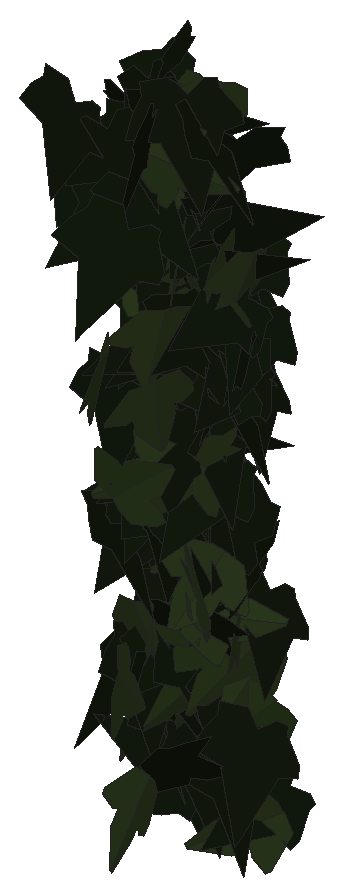
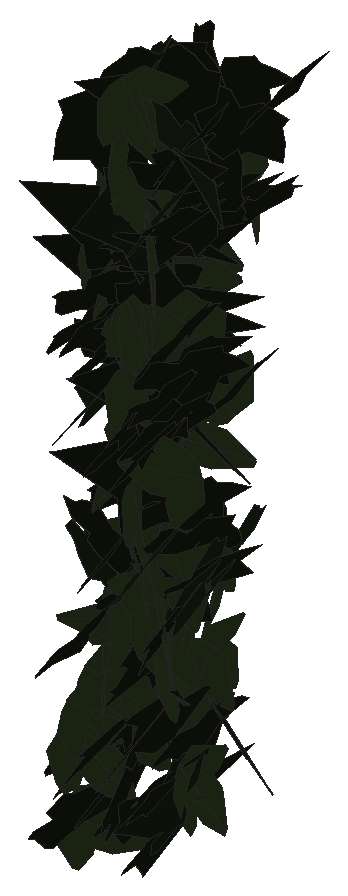
# SketchUp Ruby script. Lengths in inches.
U = 1.inch
M = Sketchup.active_model
def pt(a) = Geom::Point3d.new(a.map { |v| v * U })
def face(e, loops, mat)
  f = e.add_face(loops[0].map { |a| pt(a) })
  loops[1..].each { |l| e.add_face(l.map { |a| pt(a) }).erase! }
  f.material = f.back_material = mat if mat
  f
end
# faces: each face lists its corners as indices into pts; further lists are holes
def faces(e, pts, list, mat = nil) = list.each { |f| face(e, (f[0].is_a?(Array) ? f : [f]).map { |l| l.map { |i| pts[i] } }, mat) }
# xy, xz, yz: faces in a plane at the given z, y or x. An outline is a flat list of corners, or four numbers for a rectangle; further outlines are holes
def ring(l) = l.size == 4 ? [[l[0], l[1]], [l[2], l[1]], [l[2], l[3]], [l[0], l[3]]] : l.each_slice(2).to_a
def flat(e, list, mat, &to3) = list.each { |f| face(e, (f[0].is_a?(Array) ? f : [f]).map { |l| ring(l).map { |u, v| to3.(u, v) } }, mat) }
def xy(e, z, list, mat = nil) = flat(e, list, mat) { |x, y| [x, y, z] }
def xz(e, y, list, mat = nil) = flat(e, list, mat) { |x, z| [x, y, z] }
def yz(e, x, list, mat = nil) = flat(e, list, mat) { |y, z| [x, y, z] }
def lines(e, pts, list) = list.each { |a, b| e.add_line(pt(pts[a]), pt(pts[b])) }
# prism: a flat outline (further loops are holes) pulled along v
def prism(e, loops, v, mat = nil)
  f = face(e, loops, mat); d = Geom::Vector3d.new(v.map { |x| x * U })
  f.pushpull(f.normal.samedirection?(d) ? d.length : -d.length)
end
def box(e, o, s, mat = nil) = prism(e, [[o, [o[0] + s[0], o[1], o[2]], [o[0] + s[0], o[1] + s[1], o[2]], [o[0], o[1] + s[1], o[2]]]], [0, 0, s[2]], mat)
def at(x, y, z, deg = 0) = Geom::Transformation.translation(pt([x, y, z])) * Geom::Transformation.rotation(ORIGIN, Z_AXIS, deg.degrees)
def axes(o, x, y, z) = Geom::Transformation.new([*x, 0, *y, 0, *z, 0, *pt(o).to_a, 1])
def part(name) = M.definitions.add(name)
# library, detail: a bought-in or finely detailed component or shape, given as its bounding box
def library(name, o, s) = part(name).tap { |d| box(d.entities, o, s) }
def detail(e, o, s) = box(e.add_group.entities, o, s)
def put(e, d, t, mat = nil) = e.add_instance(d, t).tap { |i| i.material = mat if mat }
def group(e, t, mat = nil) = e.add_group.tap { |g| g.transformation = t; g.material = mat if mat }.entities
root = M.entities
M.materials.add("efeu1").color = [18, 25, 13]
M.materials.add("efeu2").color = [43, 57, 29]
c1 = part("ivyleaf_9")
p = [[1.54,2.16,1.25],[1.36,2.04,1.19],[-0.21,0.99,0.68],[-0.71,1.11,0.82],[-0.85,0.86,0.67],[-0.8,0.17,0.21],
  [-0.9,-0.01,0.1],[-0.67,-0.16,-0.02],[-0.08,-0.08,-0.05],[-0.03,-0.6,-0.4],[0.65,-0.88,-0.66],[0.83,-0.6,-0.49],
  [1.29,-0.42,-0.43],[1.8125,-0.07,-0.26],[1.21,0.44,0.15]]
faces(c1.entities,p,[[0,1,2,3,4,5,6,7,8,9,10,11,12,13,14]],"efeu1")
c2 = part("ivyleaf_10")
p = [[0,0.5,-0.03],[-0.0625,2.02,-0.43],[-0.19,2.01,-0.46],[-0.54,1.05,-0.29],[-0.52,0.625,-0.18],[-0.83,0.76,-0.28],
  [-1.16,0.64,-0.33],[-1.15,0.33,-0.24],[-0.77,-0.39,0.02],[-0.3,-0.51,0.16],[0.04,-0.48,0.23],[-0.02,2.01,-0.4375],
  [-0.06,2.01,-0.43],[0.04,-0.49,0.23],[0.67,-0.49,0.14],[1.38,0.36,-0.2],[1.375,0.51,-0.24],[0.81,0.65,-0.19],
  [0.62,0.59,-0.15],[0.6,1.09,-0.28],[0.5,1.23,-0.31]]
faces(c2.entities,p,[[0,1,2,3,4,5,6,7,8,9,10],[11,12,0,13,14,15,16,17,18,19,20]],"efeu2")
put(root,c1,axes([20.29,222.73,225.05],[-0.44668,0.13487,-0.17969],[0.17254,-0.05023,-0.46659],[-0.14391,-0.47884,-0.00167]))
put(root,c2,axes([20.2,223.32,224.3125],[0.0873,-0.42778,0.24369],[0.0352,-0.24144,-0.43643],[0.49106,0.09336,-0.01204]))
put(root,c1,axes([20.49,223.13,233.26],[-0.21677,0.41823,0.1676],[-0.1139,0.12909,-0.46943],[-0.43593,-0.2417,0.03931]))
put(root,c1,axes([19.875,223.24,232.43],[0.43086,-0.00057,-0.25369],[0.25367,0.00712,0.43082],[0.00312,-0.49995,0.00642]))
put(root,c1,axes([20.11,221.8,233.26],[-0.04545,-0.45299,0.20672],[0.01767,-0.20892,-0.45392],[0.49762,-0.03395,0.035]))
put(root,c1,axes([20.05,222.28,232.04],[0.12078,-0.44649,-0.18989],[0.02906,0.20199,-0.45646],[0.48432,0.09923,0.07474]))
put(root,c1,axes([20.05,223.34,232.34],[0.0508,-0.42895,-0.25183],[0.08226,0.2569,-0.42099],[0.49056,0.00134,0.09667]))
put(root,c1,axes([20.17,223.11,232.35],[-0.04111,-0.49708,0.03489],[0.00283,-0.03525,-0.49875],[0.4983,-0.04081,0.00571]))
put(root,c1,axes([20.24,223.48,230.2],[-0.22662,-0.43652,-0.08994],[0.05094,0.07487,-0.49173],[0.44277,-0.23204,0.01054]))
put(root,c1,axes([20.52,223.53,232.92],[-0.45123,-0.20098,0.07745],[-0.07015,-0.03286,-0.49396],[0.20364,-0.45665,0.00146]))
put(root,c1,axes([20.33,223.09,227.02],[-0.22902,-0.39992,0.19395],[-0.01831,-0.20951,-0.45362],[0.44409,-0.21488,0.08131]))
put(root,c1,axes([20.08,223.25,227.1],[0.33827,-0.3615,0.06994],[0.04312,-0.05543,-0.49504],[0.36567,0.34095,-0.00632]))
put(root,c1,axes([20.4,223.26,230.13],[-0.22306,-0.43913,0.08605],[-0.01732,-0.08761,-0.49196],[0.44715,-0.22246,0.02387]))
put(root,c1,axes([20.27,223.13,224.95],[0.02355,-0.49943,0.0041],[-0.00019,-0.00411,-0.49998],[0.49944,0.02355,-0.00039]))
put(root,c2,axes([20.45,222.8,225.63],[-0.49195,0.05295,-0.07198],[0.07158,-0.00756,-0.49479],[-0.05349,-0.49713,-0.00015]))
put(root,c1,axes([20.2,222.43,227.17],[0.27052,-0.41736,0.05129],[0.02789,-0.04304,-0.49736],[0.41957,0.27196,-0.00001]))
put(root,c1,axes([20.32,223.51,230.55],[0.06697,-0.49321,0.04756],[-0.00058,-0.04807,-0.49768],[0.49549,0.0666,-0.00701]))
put(root,c1,axes([20.3125,223.36,226.71],[0.22358,-0.42503,-0.13914],[-0.06412,0.12349,-0.48025],[0.44261,0.23259,0.00071]))
put(root,c2,axes([20.62,223.09,227.19],[-0.20746,-0.44081,0.11246],[-0.02499,-0.11237,-0.48657],[0.45424,-0.20751,0.02459]))
put(root,c1,axes([20.61,222.25,231.8],[-0.30428,-0.29383,0.2666],[-0.07992,-0.2837,-0.40389],[0.38862,-0.28841,0.12568]))
put(root,c1,axes([20.22,223.51,224.11],[0.37611,-0.31835,0.08484],[0.07216,-0.04603,-0.49262],[0.32146,0.3828,0.01132]))
put(root,c2,axes([20.6,223.43,226.68],[0.2624,-0.40206,-0.1396],[-0.05719,0.12921,-0.47962],[0.42175,0.26768,0.02182]))
put(root,c1,axes([20.4,223.53,229.35],[0.04058,-0.48082,-0.13102],[-0.01285,0.1304,-0.48253],[0.49819,0.04253,-0.00178]))
put(root,c2,axes([20.51,223.37,225.8],[0.12563,-0.34858,0.33572],[0.11424,-0.31568,-0.37053],[0.47028,0.16981,0.00033]))
put(root,c1,axes([20.37,223.6,223.66],[0.11462,-0.48487,-0.04201],[-0.00503,0.04198,-0.49821],[0.48666,0.11463,0.00474]))
put(root,c2,axes([20.22,223.46,228.64],[-0.10493,-0.00037,-0.48887],[0.47648,-0.11194,-0.10218],[-0.10937,-0.48731,0.02385]))
put(root,c1,axes([20.38,223.02,233.125],[0.23547,-0.41776,-0.14152],[-0.05007,0.13407,-0.47908],[0.43823,0.23979,0.0213]))
put(root,c1,axes([20.55,223.5,229.65],[-0.16069,-0.46395,0.0945],[-0.01372,-0.09519,-0.49066],[0.47328,-0.16028,0.01786]))
put(root,c1,axes([20.44,223.4,224.24],[0.06464,-0.49436,-0.03782],[-0.00656,0.03728,-0.49857],[0.49576,0.06496,-0.00167]))
put(root,c1,axes([20.48,223.05,227.53],[-0.05187,-0.44356,-0.22487],[0.03363,0.22245,-0.44653],[0.49616,-0.06145,0.00676]))
put(root,c1,axes([20.47,223.18,225.25],[0.0926,-0.35564,-0.33904],[-0.01107,0.34341,-0.36324],[0.49123,0.07478,0.05573]))
put(root,c1,axes([20.49,222.27,229.17],[0.00213,-0.47226,0.1642],[0.0331,-0.16371,-0.47128],[0.4989,0.01287,0.03057]))
put(root,c1,axes([20.67,222.99,227.93],[-0.24653,-0.43417,0.02685],[-0.01024,-0.02506,-0.49927],[0.43488,-0.24672,0.00347]))
put(root,c1,axes([20.45,223.53,232.3],[0.14506,-0.4604,0.13033],[0.05425,-0.11949,-0.48247],[0.47541,0.15411,0.01528]))
put(root,c1,axes([20.47,223.33,229.18],[0.25083,-0.36174,-0.23713],[-0.0305,0.25865,-0.42682],[0.43146,0.22858,0.10768]))
put(root,c1,axes([21.0625,223.14,230.5625],[-0.24069,-0.02118,0.43775],[-0.42615,-0.10527,-0.2394],[0.10231,-0.48833,0.03262]))
put(root,c1,axes([20.94,223.04,223.5],[-0.11205,-0.4737,-0.11426],[-0.02701,-0.11102,0.48677],[-0.48653,0.11525,-0.00071]))
put(root,c1,axes([20.58,221.92,232.98],[-0.16085,-0.21942,-0.4195],[0.23547,0.34729,-0.27193],[0.41071,-0.28504,-0.00839]))
put(root,c1,axes([20.56,223.74,227.4],[0.10873,-0.45678,0.17185],[0.06527,-0.16087,-0.46889],[0.48365,0.1244,0.02464]))
put(root,c2,axes([20.84,223.34,231.77],[0.28715,-0.38121,-0.14906],[-0.0303,0.16179,-0.47213],[0.4082,0.28018,0.06981]))
put(root,c2,axes([20.59,222.85,230.6],[0.35304,0.238,0.26214],[0.21125,0.15549,-0.42567],[-0.28414,0.41131,0.00923]))
put(root,c2,axes([20.99,223.39,229.68],[-0.24606,-0.34879,0.26039],[-0.06077,-0.26866,-0.41729],[0.431,-0.23701,0.08982]))
put(root,c2,axes([20.91,222.85,229.53],[0.24974,-0.42667,-0.07474],[-0.02391,0.07256,-0.49413],[0.4325,0.25038,0.01584]))
put(root,c2,axes([20.95,223.42,228.01],[0.086,-0.49226,-0.01685],[-0.00304,0.01657,-0.49972],[0.49254,0.08606,-0.00014]))
put(root,c2,axes([20.99,223.33,226.43],[-0.16771,-0.44434,0.15633],[-0.01547,-0.16066,-0.47323],[0.47078,-0.16357,0.04014]))
put(root,c2,axes([20.9,223.1875,230.375],[-0.47866,-0.0833,-0.11808],[0.11963,0.00075,-0.48548],[0.08106,-0.49301,0.01921]))
put(root,c2,axes([21,223.25,230.54],[-0.21562,-0.45026,0.02788],[0.00887,-0.03513,-0.49869],[0.45103,-0.21456,0.02313]))
put(root,c2,axes([21.07,222.76,227.2],[-0.23237,0.28162,0.3416],[-0.203,0.27508,-0.36486],[-0.39344,-0.30826,-0.0135]))
put(root,c2,axes([20.77,223.24,226.65],[-0.27371,-0.15378,-0.38914],[0.34516,0.17987,-0.31386],[0.23652,-0.44045,0.00769]))
put(root,c2,axes([20.96,223.19,224.73],[0.02766,-0.10487,0.4881],[0.09389,-0.47903,-0.10824],[0.49033,0.09764,-0.0068]))
put(root,c1,axes([20.74,222.82,227.03],[0.07396,-0.38374,0.31189],[0.09534,-0.29838,-0.38972],[0.48522,0.11712,0.02903]))
put(root,c1,axes([21.26,223.25,231.46],[-0.43761,-0.07431,0.23016],[-0.18957,-0.19011,-0.42181],[0.1502,-0.45644,0.13821]))
put(root,c2,axes([21.01,223.39,230.55],[0.05816,-0.47589,0.14192],[0.03381,-0.13877,-0.47917],[0.49545,0.06533,0.01604]))
put(root,c1,axes([20.84,222.77,227.66],[0.00945,-0.41961,-0.27174],[0.03273,0.27172,-0.41845],[0.49884,-0.00988,0.0326]))
put(root,c1,axes([20.83,223.26,225.15],[0.13519,-0.47753,-0.06074],[-0.00266,0.06234,-0.49609],[0.48137,0.13445,0.01432]))
put(root,c1,axes([20.84,223.31,229.37],[0.14141,-0.47181,-0.08603],[-0.01045,0.08664,-0.49232],[0.47947,0.14104,0.01464]))
put(root,c1,axes([21.45,222.77,231.53],[-0.33871,0.1452,0.33792],[-0.3294,0.0846,-0.36652],[-0.16361,-0.47091,0.03835]))
put(root,c2,axes([21.33,222.22,228.25],[-0.09887,-0.10109,0.47959],[-0.30836,-0.36746,-0.14102],[0.38097,-0.32366,0.01032]))
put(root,c1,axes([21.05,223.78,223.7],[-0.10679,0.02546,0.4878],[-0.14758,-0.47767,-0.00738],[0.46563,-0.14555,0.10954]))
put(root,c1,axes([21.29,222.64,230.1],[-0.32505,-0.21491,0.31329],[-0.26578,-0.166,-0.38963],[0.27148,-0.41983,-0.00632]))
put(root,c2,axes([21.08,223.37,227.33],[0.30731,-0.39385,-0.02103],[-0.01063,0.01837,-0.49955],[0.39427,0.30748,0.00292]))
put(root,c1,axes([20.85,223.64,224.7],[0.13042,-0.47201,0.10099],[0.02032,-0.09915,-0.48965],[0.48226,0.13183,-0.00668]))
put(root,c2,axes([21.11,222.81,230.21],[-0.01684,-0.37857,0.3262],[0.02601,-0.3266,-0.37769],[0.49904,0.00425,0.0307]))
put(root,c1,axes([20.94,223.11,226.57],[-0.13405,-0.3772,-0.29958],[0.11784,0.27584,-0.40003],[0.46706,-0.17785,0.01495]))
put(root,c2,axes([21.01,222.97,232],[0.36093,0.3454,0.02077],[0.01528,0.01407,-0.49957],[-0.34569,0.36125,-0.0004]))
put(root,c2,axes([20.97,222.83,231.22],[0.30802,-0.3005,0.2546],[0.1923,-0.16732,-0.43014],[0.34372,0.36291,0.01249]))
put(root,c1,axes([20.7,223.24,229.55],[0.18359,-0.01293,-0.4649],[0.38196,0.28935,0.14279],[0.26534,-0.40757,0.11612]))
put(root,c2,axes([21.15,222.95,233.23],[0.41391,-0.2799,-0.01825],[-0.01475,0.01078,-0.49967],[0.28011,0.41417,0.00067]))
put(root,c1,axes([20.99,223.33,223.79],[0.03703,-0.49287,-0.07552],[0,0.07573,-0.49423],[0.49863,0.0366,0.00561]))
put(root,c2,axes([21.27,222.09,230.42],[-0.1936,-0.45507,0.07369],[-0.01138,-0.07518,-0.49418],[0.46086,-0.19303,0.01875]))
put(root,c1,axes([20.83,223.09,228.28],[0.21602,0.2233,-0.39175],[0.27614,0.2779,0.31067],[0.35648,-0.35058,-0.00326]))
put(root,c1,axes([20.99,221.87,232.42],[0.19804,-0.38297,-0.25321],[0.00357,0.27704,-0.41622],[0.45909,0.16305,0.11247]))
put(root,c1,axes([21.57,222.16,228.64],[-0.47501,0.13201,0.08332],[-0.08209,0.01578,-0.49296],[-0.13278,-0.482,0.00668]))
put(root,c1,axes([21.375,222.92,231.67],[-0.21458,0.35337,-0.28122],[-0.14436,0.24135,0.41341],[0.42792,0.25862,-0.00155]))
put(root,c1,axes([21.23,222.59,226.06],[0.45654,0.18578,-0.08401],[-0.07975,-0.0269,-0.49287],[-0.18765,0.46342,0.00507]))
put(root,c1,axes([21.53,222.55,230.37],[0.0097,0.04092,-0.49823],[-0.08364,-0.49117,-0.04197],[-0.49286,0.08416,-0.00268]))
put(root,c2,axes([21.45,222.97,233.34],[-0.22124,-0.40203,0.19855],[-0.04439,-0.20068,-0.4558],[0.44619,-0.21931,0.0531]))
put(root,c1,axes([20.95,222.43,233.07],[0.22696,-0.00671,0.44547],[0.44446,-0.03116,-0.22691],[0.0308,0.49898,-0.00817]))
put(root,c2,axes([21.49,222.64,226.11],[-0.0655,0.30667,-0.38944],[-0.06919,0.38333,0.31349],[0.49084,0.09496,-0.00778]))
put(root,c1,axes([21.3125,221.83,233.39],[-0.17104,0.1155,-0.45542],[0.36844,-0.26777,-0.20628],[-0.29154,-0.40615,0.00649]))
put(root,c1,axes([21.44,223.1,228.01],[-0.27559,-0.40236,0.11023],[-0.06539,-0.08882,-0.48768],[0.41203,-0.28322,-0.00367]))
put(root,c1,axes([21.22,223.13,226.96],[0.02763,-0.35725,0.34872],[0.06238,-0.34405,-0.35741],[0.49532,0.06325,0.02556]))
put(root,c1,axes([21.47,223.74,230.96],[-0.31233,-0.37873,0.09495],[-0.02968,-0.0982,-0.48936],[0.38932,-0.31132,0.03886]))
put(root,c1,axes([21.22,223.375,224.76],[0.25035,-0.34348,-0.26334],[-0.05198,0.27815,-0.41222],[0.42968,0.23378,0.10356]))
put(root,c2,axes([21.74,223.58,224.42],[-0.28941,-0.18583,0.36292],[-0.30686,-0.19379,-0.34393],[0.26848,-0.4218,-0.00188]))
put(root,c2,axes([21.6,223.33,225.26],[-0.09208,-0.32123,0.37193],[-0.08222,-0.363,-0.33388],[0.48452,-0.12265,0.01403]))
put(root,c1,axes([21.31,223.11,228.6875],[0.06239,-0.48935,-0.08153],[-0.01049,0.08085,-0.49331],[0.49598,0.06327,-0.00018]))
put(root,c1,axes([21.89,223.12,227.08],[-0.24533,0.16518,0.40315],[-0.33677,0.22163,-0.29575],[-0.2764,-0.41665,0.00251]))
put(root,c1,axes([21.38,223.53,227.11],[-0.03233,-0.40478,0.29173],[0.00839,-0.29274,-0.40525],[0.49888,-0.0213,0.02572]))
put(root,c2,axes([21.55,220.93,225.92],[0.1793,-0.33755,-0.32235],[0.02802,0.35248,-0.35352],[0.46591,0.1087,0.14531]))
put(root,c2,axes([21.5,222.79,230.57],[-0.4714,0.12226,-0.11328],[0.10993,-0.02735,-0.487],[-0.12528,-0.48405,-0.00109]))
put(root,c2,axes([21.68,222.74,230.86],[-0.02296,0.10943,0.48734],[-0.2248,0.43338,-0.10791],[-0.44602,-0.22406,0.0293]))
put(root,c2,axes([21.57,223.77,225.04],[-0.10958,-0.28783,0.39389],[0.07684,-0.40885,-0.27738],[0.48176,-0.00026,0.13384]))
put(root,c2,axes([21.6,222.64,228.24],[-0.01322,0.24592,0.43514],[-0.1106,0.42307,-0.24245],[-0.48744,-0.10266,0.04321]))
put(root,c2,axes([21.34,221.25,228.38],[-0.33168,-0.0938,0.3622],[0.34738,0.10261,0.34467],[-0.13899,0.48028,-0.0029]))
put(root,c1,axes([21.47,221.63,224.25],[0.27517,0.31701,0.27163],[0.1691,0.21281,-0.41966],[-0.38169,0.32282,0.00991]))
put(root,c1,axes([21.49,222.35,233.6],[-0.15363,-0.41138,-0.2391],[0.08602,0.2231,-0.43912],[0.46797,-0.17606,0.00222]))
put(root,c2,axes([21.6,223.16,232.07],[-0.44165,0.20024,0.12185],[0.10163,-0.07063,0.48444],[0.21122,0.45268,0.02169]))
put(root,c2,axes([21.64,223.17,225.83],[0.24023,-0.39085,-0.19882],[-0.00739,0.22305,-0.44743],[0.43845,0.21791,0.10139]))
put(root,c1,axes([21.27,222.86,230.85],[0.24399,0.29745,-0.31937],[0.19948,0.24942,0.3847],[0.38817,-0.31514,0.00304]))
put(root,c2,axes([21.34,222.06,232.84],[-0.16016,-0.06264,-0.46949],[0.46844,0.05239,-0.16679],[0.07009,-0.49329,0.0419]))
put(root,c1,axes([21.53,223.37,230.37],[-0.02656,-0.49929,0.00043],[0.00126,-0.0005,-0.5],[0.49929,-0.02656,0.00128]))
put(root,c2,axes([21.76,222.51,226.92],[0.43903,0.11279,-0.21101],[-0.20705,-0.0419,-0.45318],[-0.11991,0.48531,0.00992]))
put(root,c1,axes([22.07,222.77,229.55],[-0.34705,0.0374,0.35799],[-0.35993,-0.0397,-0.34479],[0.00263,-0.49702,0.05449]))
put(root,c2,axes([21.36,222.87,225.98],[0.00079,-0.11212,-0.48727],[0.4752,0.15172,-0.03414],[0.15551,-0.46304,0.1068]))
put(root,c1,axes([21.55,223.14,223.73],[0.11006,-0.48353,0.06395],[0.01071,-0.06314,-0.49588],[0.48762,0.11052,-0.00354]))
put(root,c1,axes([21.9,222.81,232.92],[0.08839,0.40092,-0.28539],[-0.06659,-0.27755,-0.41053],[-0.4876,0.11058,0.00433]))
put(root,c2,axes([22.03,223.2,223.08],[0.13838,0.14676,-0.45751],[-0.41883,-0.19646,-0.1897],[-0.23544,0.43574,0.06856]))
put(root,c1,axes([21.84,220.66,232.54],[-0.37851,-0.32098,-0.06084],[0.04403,0.04214,-0.49627],[0.32371,-0.38105,-0.00364]))
put(root,c1,axes([21.58,223.55,229.24],[0.08127,-0.4748,0.13403],[0.04322,-0.12846,-0.48128],[0.49145,0.08981,0.02016]))
put(root,c1,axes([21.47,223,231.4375],[0.12942,-0.0111,0.48283],[0.47735,-0.073,-0.12963],[0.07337,0.49452,-0.0083]))
put(root,c1,axes([22.11,222.96,226.87],[-0.36666,0.33808,-0.03557],[0.02524,-0.02511,-0.49873],[-0.33901,-0.36752,0.00135]))
put(root,c1,axes([21.9,222.97,230.61],[-0.24929,-0.28172,0.32938],[-0.0848,-0.34093,-0.35578],[0.42505,-0.23324,0.1222]))
put(root,c1,axes([21.69,223.74,225.96],[0.01024,-0.48738,0.11114],[0.02782,-0.11044,-0.48686],[0.49912,0.01615,0.02486]))
put(root,c1,axes([21.62,222.48,233.3],[0.31564,-0.38607,-0.03637],[-0.02005,0.03059,-0.49866],[0.38726,0.31625,0.00383]))
put(root,c1,axes([21.98,223.71,223.3125],[-0.24441,-0.31458,0.30216],[-0.16993,-0.25033,-0.39807],[0.40173,-0.29728,0.01545]))
put(root,c2,axes([21.92,222.98,231.06],[0.018,-0.47252,0.16249],[0.02861,-0.16136,-0.47238],[0.49886,0.02631,0.02123]))
put(root,c1,axes([21.84,223.12,229.63],[-0.14184,-0.36544,0.31038],[-0.04371,-0.31247,-0.38788],[0.47746,-0.13717,0.05669]))
put(root,c2,axes([21.9375,220.0625,230.97],[0.20442,-0.44752,-0.08909],[-0.02139,0.08811,-0.49171],[0.4558,0.20484,0.01688]))
put(root,c2,axes([21.88,220.9,224.41],[-0.00679,-0.34817,0.35879],[0.15772,-0.34199,-0.32889],[0.47443,0.10871,0.11447]))
put(root,c1,axes([22.01,222.84,230.1],[-0.38919,0.1543,-0.27335],[0.25682,-0.09383,-0.41862],[-0.18048,-0.46625,-0.00622]))
put(root,c1,axes([21.87,223.25,224.24],[-0.12953,-0.48289,0.00629],[-0.00109,-0.00622,-0.49996],[0.48293,-0.12953,0.00056]))
put(root,c2,axes([22,221.05,230.13],[-0.19636,-0.44933,-0.09772],[0.03515,0.09128,-0.49034],[0.45848,-0.19944,-0.00425]))
put(root,c1,axes([21.86,223.35,230.22],[-0.10962,-0.46811,0.13731],[-0.00058,-0.14061,-0.47982],[0.48783,-0.10536,0.03029]))
put(root,c1,axes([21.67,222.97,229.3],[0.23832,-0.41249,0.15184],[0.09059,-0.12292,-0.47611],[0.43011,0.25445,0.01615]))
put(root,c2,axes([22.03,221.95,226.69],[-0.37882,0.32093,0.05912],[0.04054,-0.04359,0.49644],[0.32381,0.38092,0.007]))
